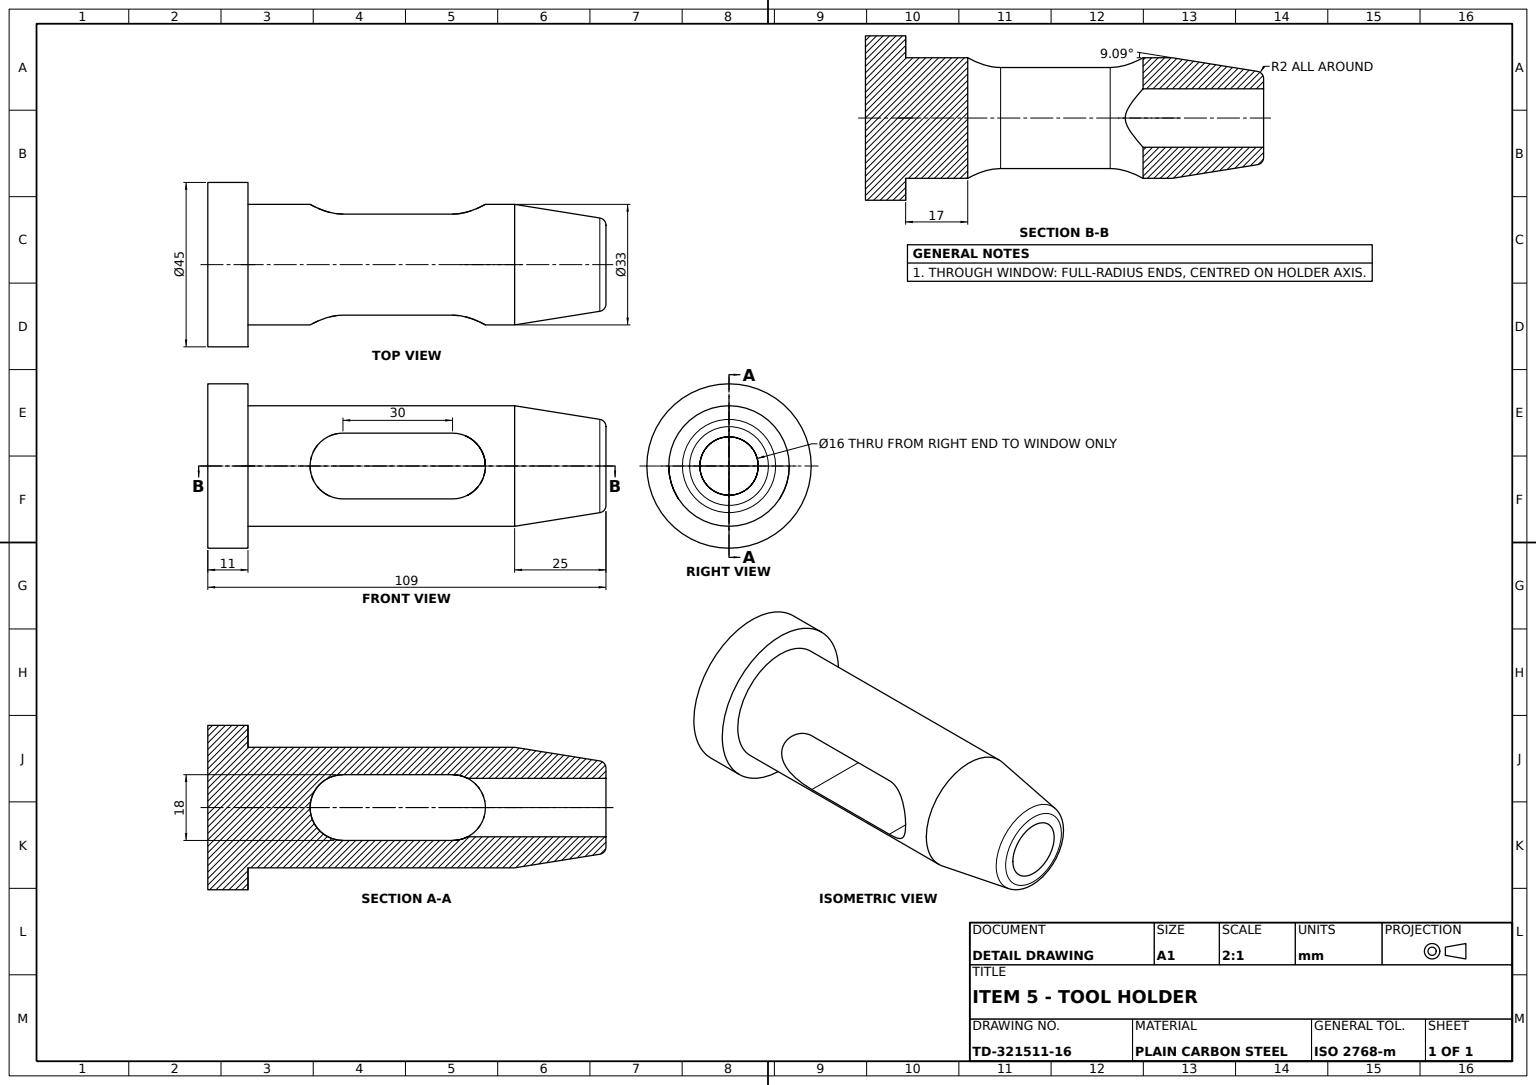
ISO-10303-21;
HEADER;
FILE_DESCRIPTION((''),'2;1');
FILE_NAME('','',(''),(''),'','','');
FILE_SCHEMA(('AUTOMOTIVE_DESIGN'));
ENDSEC;
DATA;
#1=APPLICATION_CONTEXT('');
#2=PRODUCT_CONTEXT('',#1,'mechanical');
#3=PRODUCT('','','',(#2));
#4=PRODUCT_DEFINITION_FORMATION('','',#3);
#5=PRODUCT_DEFINITION_CONTEXT('',#1,'design');
#6=PRODUCT_DEFINITION('','',#4,#5);
#7=PRODUCT_DEFINITION_SHAPE('','',#6);
#8=(LENGTH_UNIT()NAMED_UNIT(*)SI_UNIT(.MILLI.,.METRE.));
#9=(NAMED_UNIT(*)PLANE_ANGLE_UNIT()SI_UNIT($,.RADIAN.));
#10=(NAMED_UNIT(*)SI_UNIT($,.STERADIAN.)SOLID_ANGLE_UNIT());
#11=UNCERTAINTY_MEASURE_WITH_UNIT(LENGTH_MEASURE(1.E-05),#8,'distance_accuracy_value','');
#12=(GEOMETRIC_REPRESENTATION_CONTEXT(3)GLOBAL_UNCERTAINTY_ASSIGNED_CONTEXT((#11))GLOBAL_UNIT_ASSIGNED_CONTEXT((#8,#9,#10))REPRESENTATION_CONTEXT('',''));
#13=CARTESIAN_POINT('',(109.,0.,-10.794562));
#14=VERTEX_POINT('',#13);
#15=CARTESIAN_POINT('',(107.315981,0.,-12.769443));
#16=VERTEX_POINT('',#15);
#17=CARTESIAN_POINT('',(107.,0.,-10.794562));
#18=DIRECTION('',(0.,1.,0.));
#19=DIRECTION('',(0.,0.,1.));
#20=AXIS2_PLACEMENT_3D('',#17,#18,#19);
#21=CIRCLE('',#20,2.);
#22=EDGE_CURVE('',#14,#16,#21,.T.);
#23=ORIENTED_EDGE('',*,*,#22,.T.);
#24=CARTESIAN_POINT('',(107.315981,0.,12.769443));
#25=VERTEX_POINT('',#24);
#26=CARTESIAN_POINT('',(107.315981,0.,0.));
#27=DIRECTION('',(-1.,0.,0.));
#28=DIRECTION('',(0.,0.,-1.));
#29=AXIS2_PLACEMENT_3D('',#26,#27,#28);
#30=CIRCLE('',#29,12.769443);
#31=EDGE_CURVE('',#25,#16,#30,.T.);
#32=ORIENTED_EDGE('',*,*,#31,.F.);
#33=CARTESIAN_POINT('',(109.,0.,10.794562));
#34=VERTEX_POINT('',#33);
#35=CARTESIAN_POINT('',(107.,0.,10.794562));
#36=DIRECTION('',(0.,-1.,0.));
#37=AXIS2_PLACEMENT_3D('',#35,#36,#28);
#38=CIRCLE('',#37,2.);
#39=EDGE_CURVE('',#34,#25,#38,.T.);
#40=ORIENTED_EDGE('',*,*,#39,.F.);
#41=CARTESIAN_POINT('',(109.,0.,0.));
#42=DIRECTION('',(1.,0.,0.));
#43=AXIS2_PLACEMENT_3D('',#41,#42,#19);
#44=CIRCLE('',#43,10.794562);
#45=EDGE_CURVE('',#14,#34,#44,.T.);
#46=ORIENTED_EDGE('',*,*,#45,.F.);
#47=EDGE_LOOP('',(#23,#32,#40,#46));
#48=FACE_OUTER_BOUND('',#47,.T.);
#49=CARTESIAN_POINT('',(107.,0.,0.));
#50=AXIS2_PLACEMENT_3D('',#49,#27,#19);
#51=TOROIDAL_SURFACE('',#50,10.794562,2.);
#52=ADVANCED_FACE('',(#48),#51,.T.);
#53=CARTESIAN_POINT('',(67.,9.,-13.829317));
#54=VERTEX_POINT('',#53);
#55=CARTESIAN_POINT('',(37.,9.,-13.829317));
#56=VERTEX_POINT('',#55);
#57=CARTESIAN_POINT('',(-42.829787,9.,-13.829317));
#58=VECTOR('',#27,1000.);
#59=LINE('',#57,#58);
#60=EDGE_CURVE('',#54,#56,#59,.T.);
#61=ORIENTED_EDGE('',*,*,#60,.F.);
#62=CARTESIAN_POINT('',(67.,9.,13.829317));
#63=VERTEX_POINT('',#62);
#64=CARTESIAN_POINT('',(67.,9.,-22.5));
#65=VECTOR('',#19,1000.);
#66=LINE('',#64,#65);
#67=EDGE_CURVE('',#54,#63,#66,.T.);
#68=ORIENTED_EDGE('',*,*,#67,.T.);
#69=CARTESIAN_POINT('',(37.,9.,13.829317));
#70=VERTEX_POINT('',#69);
#71=CARTESIAN_POINT('',(-42.829787,9.,13.829317));
#72=VECTOR('',#42,1000.);
#73=LINE('',#71,#72);
#74=EDGE_CURVE('',#70,#63,#73,.T.);
#75=ORIENTED_EDGE('',*,*,#74,.F.);
#76=CARTESIAN_POINT('',(37.,9.,-22.5));
#77=LINE('',#76,#65);
#78=EDGE_CURVE('',#56,#70,#77,.T.);
#79=ORIENTED_EDGE('',*,*,#78,.F.);
#80=EDGE_LOOP('',(#61,#68,#75,#79));
#81=FACE_OUTER_BOUND('',#80,.T.);
#82=AXIS2_PLACEMENT_3D('',#76,#18,#19);
#83=PLANE('',#82);
#84=ADVANCED_FACE('',(#81),#83,.F.);
#85=CARTESIAN_POINT('',(11.,0.,22.5));
#86=VERTEX_POINT('',#85);
#87=CARTESIAN_POINT('',(0.,0.,22.5));
#88=VERTEX_POINT('',#87);
#89=CARTESIAN_POINT('',(-42.829787,0.,22.5));
#90=LINE('',#89,#58);
#91=EDGE_CURVE('',#86,#88,#90,.T.);
#92=ORIENTED_EDGE('',*,*,#91,.T.);
#93=CARTESIAN_POINT('',(0.,0.,-22.5));
#94=VERTEX_POINT('',#93);
#95=CARTESIAN_POINT('',(0.,0.,0.));
#96=AXIS2_PLACEMENT_3D('',#95,#27,#19);
#97=CIRCLE('',#96,22.5);
#98=EDGE_CURVE('',#94,#88,#97,.T.);
#99=ORIENTED_EDGE('',*,*,#98,.F.);
#100=CARTESIAN_POINT('',(11.,0.,-22.5));
#101=VERTEX_POINT('',#100);
#102=CARTESIAN_POINT('',(-42.829787,0.,-22.5));
#103=LINE('',#102,#58);
#104=EDGE_CURVE('',#101,#94,#103,.T.);
#105=ORIENTED_EDGE('',*,*,#104,.F.);
#106=CARTESIAN_POINT('',(11.,0.,0.));
#107=AXIS2_PLACEMENT_3D('',#106,#27,#19);
#108=CIRCLE('',#107,22.5);
#109=EDGE_CURVE('',#101,#86,#108,.T.);
#110=ORIENTED_EDGE('',*,*,#109,.T.);
#111=EDGE_LOOP('',(#92,#99,#105,#110));
#112=FACE_OUTER_BOUND('',#111,.T.);
#113=CARTESIAN_POINT('',(-42.829787,0.,0.));
#114=AXIS2_PLACEMENT_3D('',#113,#27,#19);
#115=CYLINDRICAL_SURFACE('',#114,22.5);
#116=ADVANCED_FACE('',(#112),#115,.T.);
#117=CARTESIAN_POINT('',(67.,-9.,13.829317));
#118=VERTEX_POINT('',#117);
#119=CARTESIAN_POINT('',(37.,-9.,13.829317));
#120=VERTEX_POINT('',#119);
#121=CARTESIAN_POINT('',(-42.829787,-9.,13.829317));
#122=LINE('',#121,#58);
#123=EDGE_CURVE('',#118,#120,#122,.T.);
#124=ORIENTED_EDGE('',*,*,#123,.F.);
#125=CARTESIAN_POINT('',(67.,-9.,-13.829317));
#126=VERTEX_POINT('',#125);
#127=CARTESIAN_POINT('',(67.,-9.,-22.5));
#128=LINE('',#127,#65);
#129=EDGE_CURVE('',#126,#118,#128,.T.);
#130=ORIENTED_EDGE('',*,*,#129,.F.);
#131=CARTESIAN_POINT('',(37.,-9.,-13.829317));
#132=VERTEX_POINT('',#131);
#133=CARTESIAN_POINT('',(-42.829787,-9.,-13.829317));
#134=LINE('',#133,#72);
#135=EDGE_CURVE('',#132,#126,#134,.T.);
#136=ORIENTED_EDGE('',*,*,#135,.F.);
#137=CARTESIAN_POINT('',(37.,-9.,-22.5));
#138=LINE('',#137,#65);
#139=EDGE_CURVE('',#132,#120,#138,.T.);
#140=ORIENTED_EDGE('',*,*,#139,.T.);
#141=EDGE_LOOP('',(#124,#130,#136,#140));
#142=FACE_OUTER_BOUND('',#141,.T.);
#143=AXIS2_PLACEMENT_3D('',#137,#36,#28);
#144=PLANE('',#143);
#145=ADVANCED_FACE('',(#142),#144,.F.);
#146=ORIENTED_EDGE('',*,*,#135,.T.);
#147=CARTESIAN_POINT('',(76.,0.,-16.5));
#148=VERTEX_POINT('',#147);
#149=CARTESIAN_POINT('',(67.608745,-9.,-13.829317));
#150=CARTESIAN_POINT('',(68.204136,-8.938913,-13.869585));
#151=CARTESIAN_POINT('',(69.370567,-8.702558,-14.019095));
#152=CARTESIAN_POINT('',(69.946767,-8.524146,-14.130046));
#153=CARTESIAN_POINT('',(71.028904,-8.069227,-14.39468));
#154=CARTESIAN_POINT('',(71.540157,-7.792772,-14.548404));
#155=CARTESIAN_POINT('',(72.508177,-7.14145,-14.878947));
#156=CARTESIAN_POINT('',(72.954194,-6.773387,-15.052097));
#157=CARTESIAN_POINT('',(73.564861,-6.16323,-15.307292));
#158=CARTESIAN_POINT('',(73.758993,-5.949812,-15.391775));
#159=CARTESIAN_POINT('',(74.12832,-5.501936,-15.557497));
#160=CARTESIAN_POINT('',(74.304059,-5.266458,-15.639015));
#161=CARTESIAN_POINT('',(74.791958,-4.541454,-15.870812));
#162=CARTESIAN_POINT('',(75.068713,-4.029999,-16.009872));
#163=CARTESIAN_POINT('',(75.410231,-3.217805,-16.185563));
#164=CARTESIAN_POINT('',(75.511702,-2.939521,-16.23864));
#165=CARTESIAN_POINT('',(75.688431,-2.366649,-16.331969));
#166=CARTESIAN_POINT('',(75.762616,-2.075008,-16.371651));
#167=CARTESIAN_POINT('',(75.939961,-1.197281,-16.467027));
#168=CARTESIAN_POINT('',(76.,-0.603261,-16.5));
#169=B_SPLINE_CURVE_WITH_KNOTS('',3,(#125,#149,#150,#151,#152,#153,#154,#155,#156,#157,#158,#159,#160,#161,#162,#163,#164,#165,#166,#167,#168,#147),.UNSPECIFIED.,.F.,.F.,(4,2,2,2,2,2,2,2,2,2,4),(0.,0.00179654,0.003593081,0.005389621,0.007186162,0.008084432,0.008982702,0.010779243,0.011677513,0.012575783,0.014372324),.UNSPECIFIED.);
#170=EDGE_CURVE('',#126,#148,#169,.T.);
#171=ORIENTED_EDGE('',*,*,#170,.T.);
#172=CARTESIAN_POINT('',(84.,0.,-16.5));
#173=VERTEX_POINT('',#172);
#174=CARTESIAN_POINT('',(-42.829787,0.,-16.5));
#175=LINE('',#174,#58);
#176=EDGE_CURVE('',#173,#148,#175,.T.);
#177=ORIENTED_EDGE('',*,*,#176,.F.);
#178=CARTESIAN_POINT('',(84.,0.,16.5));
#179=VERTEX_POINT('',#178);
#180=CARTESIAN_POINT('',(84.,0.,0.));
#181=AXIS2_PLACEMENT_3D('',#180,#27,#19);
#182=CIRCLE('',#181,16.5);
#183=EDGE_CURVE('',#173,#179,#182,.T.);
#184=ORIENTED_EDGE('',*,*,#183,.T.);
#185=CARTESIAN_POINT('',(76.,0.,16.5));
#186=VERTEX_POINT('',#185);
#187=CARTESIAN_POINT('',(-42.829787,0.,16.5));
#188=LINE('',#187,#58);
#189=EDGE_CURVE('',#179,#186,#188,.T.);
#190=ORIENTED_EDGE('',*,*,#189,.T.);
#191=CARTESIAN_POINT('',(76.,-0.301003,16.5));
#192=CARTESIAN_POINT('',(75.984626,-0.605798,16.4916));
#193=CARTESIAN_POINT('',(75.924121,-1.204388,16.458715));
#194=CARTESIAN_POINT('',(75.879136,-1.499868,16.434311));
#195=CARTESIAN_POINT('',(75.760581,-2.08348,16.370561));
#196=CARTESIAN_POINT('',(75.687009,-2.371611,16.331214));
#197=CARTESIAN_POINT('',(75.511256,-2.94061,16.238408));
#198=CARTESIAN_POINT('',(75.408495,-3.222513,16.184656));
#199=CARTESIAN_POINT('',(75.064128,-4.039723,16.007542));
#200=CARTESIAN_POINT('',(74.78564,-4.55228,15.8677));
#201=CARTESIAN_POINT('',(74.296702,-5.276648,15.635577));
#202=CARTESIAN_POINT('',(74.120962,-5.511434,15.554126));
#203=CARTESIAN_POINT('',(73.751604,-5.958175,15.388532));
#204=CARTESIAN_POINT('',(73.557493,-6.17105,15.304134));
#205=CARTESIAN_POINT('',(72.946994,-6.77964,15.049251));
#206=CARTESIAN_POINT('',(72.501067,-7.146844,14.876331));
#207=CARTESIAN_POINT('',(71.534185,-7.796171,14.546557));
#208=CARTESIAN_POINT('',(71.025012,-8.070838,14.39374));
#209=CARTESIAN_POINT('',(70.219751,-8.409399,14.196798));
#210=CARTESIAN_POINT('',(69.944361,-8.509905,14.13655));
#211=CARTESIAN_POINT('',(69.378428,-8.685092,14.029601));
#212=CARTESIAN_POINT('',(69.086245,-8.759986,13.982762));
#213=CARTESIAN_POINT('',(68.205376,-8.939025,13.869527));
#214=CARTESIAN_POINT('',(67.608073,-9.,13.829317));
#215=B_SPLINE_CURVE_WITH_KNOTS('',3,(#185,#191,#192,#193,#194,#195,#196,#197,#198,#199,#200,#201,#202,#203,#204,#205,#206,#207,#208,#209,#210,#211,#212,#213,#214,#117),.UNSPECIFIED.,.F.,.F.,(4,2,2,2,2,2,2,2,2,2,2,2,4),(0.014372324,0.015268727,0.016165129,0.017061532,0.017957935,0.01975074,0.020647142,0.021543545,0.02333635,0.025129156,0.026025558,0.026921961,0.028714766),.UNSPECIFIED.);
#216=EDGE_CURVE('',#186,#118,#215,.T.);
#217=ORIENTED_EDGE('',*,*,#216,.T.);
#218=ORIENTED_EDGE('',*,*,#123,.T.);
#219=CARTESIAN_POINT('',(28.,0.,16.5));
#220=VERTEX_POINT('',#219);
#221=CARTESIAN_POINT('',(36.391255,-9.,13.829317));
#222=CARTESIAN_POINT('',(35.795864,-8.938913,13.869585));
#223=CARTESIAN_POINT('',(34.629433,-8.702558,14.019095));
#224=CARTESIAN_POINT('',(34.053233,-8.524146,14.130046));
#225=CARTESIAN_POINT('',(32.971096,-8.069227,14.39468));
#226=CARTESIAN_POINT('',(32.459843,-7.792772,14.548404));
#227=CARTESIAN_POINT('',(31.491823,-7.14145,14.878947));
#228=CARTESIAN_POINT('',(31.045806,-6.773387,15.052097));
#229=CARTESIAN_POINT('',(30.435139,-6.16323,15.307292));
#230=CARTESIAN_POINT('',(30.241007,-5.949812,15.391775));
#231=CARTESIAN_POINT('',(29.87168,-5.501936,15.557497));
#232=CARTESIAN_POINT('',(29.695941,-5.266458,15.639015));
#233=CARTESIAN_POINT('',(29.208042,-4.541454,15.870812));
#234=CARTESIAN_POINT('',(28.931287,-4.029999,16.009872));
#235=CARTESIAN_POINT('',(28.589769,-3.217805,16.185563));
#236=CARTESIAN_POINT('',(28.488298,-2.939521,16.23864));
#237=CARTESIAN_POINT('',(28.311569,-2.366649,16.331969));
#238=CARTESIAN_POINT('',(28.237384,-2.075008,16.371651));
#239=CARTESIAN_POINT('',(28.060039,-1.197281,16.467027));
#240=CARTESIAN_POINT('',(28.,-0.603261,16.5));
#241=B_SPLINE_CURVE_WITH_KNOTS('',3,(#119,#221,#222,#223,#224,#225,#226,#227,#228,#229,#230,#231,#232,#233,#234,#235,#236,#237,#238,#239,#240,#219),.UNSPECIFIED.,.F.,.F.,(4,2,2,2,2,2,2,2,2,2,4),(0.,0.00179654,0.003593081,0.005389621,0.007186162,0.008084432,0.008982702,0.010779243,0.011677513,0.012575783,0.014372324),.UNSPECIFIED.);
#242=EDGE_CURVE('',#120,#220,#241,.T.);
#243=ORIENTED_EDGE('',*,*,#242,.T.);
#244=CARTESIAN_POINT('',(11.,0.,16.5));
#245=VERTEX_POINT('',#244);
#246=EDGE_CURVE('',#220,#245,#188,.T.);
#247=ORIENTED_EDGE('',*,*,#246,.T.);
#248=CARTESIAN_POINT('',(11.,0.,-16.5));
#249=VERTEX_POINT('',#248);
#250=CIRCLE('',#107,16.5);
#251=EDGE_CURVE('',#249,#245,#250,.T.);
#252=ORIENTED_EDGE('',*,*,#251,.F.);
#253=CARTESIAN_POINT('',(28.,0.,-16.5));
#254=VERTEX_POINT('',#253);
#255=EDGE_CURVE('',#254,#249,#175,.T.);
#256=ORIENTED_EDGE('',*,*,#255,.F.);
#257=CARTESIAN_POINT('',(28.,-0.301003,-16.5));
#258=CARTESIAN_POINT('',(28.015374,-0.605798,-16.4916));
#259=CARTESIAN_POINT('',(28.075879,-1.204388,-16.458715));
#260=CARTESIAN_POINT('',(28.120864,-1.499868,-16.434311));
#261=CARTESIAN_POINT('',(28.239419,-2.08348,-16.370561));
#262=CARTESIAN_POINT('',(28.312991,-2.371611,-16.331214));
#263=CARTESIAN_POINT('',(28.488744,-2.94061,-16.238408));
#264=CARTESIAN_POINT('',(28.591505,-3.222513,-16.184656));
#265=CARTESIAN_POINT('',(28.935872,-4.039723,-16.007542));
#266=CARTESIAN_POINT('',(29.21436,-4.55228,-15.8677));
#267=CARTESIAN_POINT('',(29.703298,-5.276648,-15.635577));
#268=CARTESIAN_POINT('',(29.879038,-5.511434,-15.554126));
#269=CARTESIAN_POINT('',(30.248396,-5.958175,-15.388532));
#270=CARTESIAN_POINT('',(30.442507,-6.17105,-15.304134));
#271=CARTESIAN_POINT('',(31.053006,-6.77964,-15.049251));
#272=CARTESIAN_POINT('',(31.498933,-7.146844,-14.876331));
#273=CARTESIAN_POINT('',(32.465815,-7.796171,-14.546557));
#274=CARTESIAN_POINT('',(32.974988,-8.070838,-14.39374));
#275=CARTESIAN_POINT('',(33.780249,-8.409399,-14.196798));
#276=CARTESIAN_POINT('',(34.055639,-8.509905,-14.13655));
#277=CARTESIAN_POINT('',(34.621572,-8.685092,-14.029601));
#278=CARTESIAN_POINT('',(34.913755,-8.759986,-13.982762));
#279=CARTESIAN_POINT('',(35.794624,-8.939025,-13.869527));
#280=CARTESIAN_POINT('',(36.391927,-9.,-13.829317));
#281=B_SPLINE_CURVE_WITH_KNOTS('',3,(#253,#257,#258,#259,#260,#261,#262,#263,#264,#265,#266,#267,#268,#269,#270,#271,#272,#273,#274,#275,#276,#277,#278,#279,#280,#131),.UNSPECIFIED.,.F.,.F.,(4,2,2,2,2,2,2,2,2,2,2,2,4),(0.014372324,0.015268727,0.016165129,0.017061532,0.017957935,0.01975074,0.020647142,0.021543545,0.02333635,0.025129156,0.026025558,0.026921961,0.028714766),.UNSPECIFIED.);
#282=EDGE_CURVE('',#254,#132,#281,.T.);
#283=ORIENTED_EDGE('',*,*,#282,.T.);
#284=EDGE_LOOP('',(#146,#171,#177,#184,#190,#217,#218,#243,#247,#252,#256,#283));
#285=FACE_OUTER_BOUND('',#284,.T.);
#286=CYLINDRICAL_SURFACE('',#114,16.5);
#287=ADVANCED_FACE('',(#285),#286,.T.);
#288=ORIENTED_EDGE('',*,*,#183,.F.);
#289=CARTESIAN_POINT('',(109.,0.,-12.5));
#290=DIRECTION('',(-0.987440632,0.,-0.157990501));
#291=VECTOR('',#290,1000.);
#292=LINE('',#289,#291);
#293=EDGE_CURVE('',#16,#173,#292,.T.);
#294=ORIENTED_EDGE('',*,*,#293,.F.);
#295=EDGE_CURVE('',#16,#25,#30,.T.);
#296=ORIENTED_EDGE('',*,*,#295,.T.);
#297=CARTESIAN_POINT('',(109.,0.,12.5));
#298=DIRECTION('',(-0.987440632,0.,0.157990501));
#299=VECTOR('',#298,1000.);
#300=LINE('',#297,#299);
#301=EDGE_CURVE('',#25,#179,#300,.T.);
#302=ORIENTED_EDGE('',*,*,#301,.T.);
#303=EDGE_LOOP('',(#288,#294,#296,#302));
#304=FACE_OUTER_BOUND('',#303,.T.);
#305=AXIS2_PLACEMENT_3D('',#41,#27,#19);
#306=CONICAL_SURFACE('',#305,12.5,0.158655262);
#307=ADVANCED_FACE('',(#304),#306,.T.);
#308=EDGE_CURVE('',#88,#94,#97,.T.);
#309=ORIENTED_EDGE('',*,*,#308,.T.);
#310=ORIENTED_EDGE('',*,*,#98,.T.);
#311=EDGE_LOOP('',(#309,#310));
#312=FACE_OUTER_BOUND('',#311,.T.);
#313=AXIS2_PLACEMENT_3D('',#95,#42,#28);
#314=PLANE('',#313);
#315=ADVANCED_FACE('',(#312),#314,.F.);
#316=CARTESIAN_POINT('',(76.,0.,8.));
#317=VERTEX_POINT('',#316);
#318=CARTESIAN_POINT('',(109.,0.,8.));
#319=VERTEX_POINT('',#318);
#320=CARTESIAN_POINT('',(-0.001,0.,8.));
#321=LINE('',#320,#72);
#322=EDGE_CURVE('',#317,#319,#321,.T.);
#323=ORIENTED_EDGE('',*,*,#322,.F.);
#324=CARTESIAN_POINT('',(76.,0.,-8.));
#325=VERTEX_POINT('',#324);
#326=CARTESIAN_POINT('',(76.,0.283229,8.));
#327=CARTESIAN_POINT('',(75.98643,0.570141,7.984743));
#328=CARTESIAN_POINT('',(75.932459,1.136736,7.923952));
#329=CARTESIAN_POINT('',(75.892481,1.41449,7.878894));
#330=CARTESIAN_POINT('',(75.788444,1.959657,7.761282));
#331=CARTESIAN_POINT('',(75.724377,2.227066,7.688721));
#332=CARTESIAN_POINT('',(75.573303,2.751916,7.516862));
#333=CARTESIAN_POINT('',(75.486786,3.007241,7.418113));
#334=CARTESIAN_POINT('',(75.296896,3.497221,7.200094));
#335=CARTESIAN_POINT('',(75.193148,3.733175,7.0804));
#336=CARTESIAN_POINT('',(74.969998,4.188486,6.820942));
#337=CARTESIAN_POINT('',(74.849921,4.408881,6.680382));
#338=CARTESIAN_POINT('',(74.474441,5.036934,6.236364));
#339=CARTESIAN_POINT('',(74.204096,5.412659,5.911262));
#340=CARTESIAN_POINT('',(73.779744,5.923179,5.38293));
#341=CARTESIAN_POINT('',(73.635127,6.084405,5.199952));
#342=CARTESIAN_POINT('',(73.34149,6.389866,4.819657));
#343=CARTESIAN_POINT('',(73.192093,6.534364,4.621807));
#344=CARTESIAN_POINT('',(72.747943,6.936919,4.01437));
#345=CARTESIAN_POINT('',(72.454337,7.16683,3.588994));
#346=CARTESIAN_POINT('',(72.041518,7.457306,2.906832));
#347=CARTESIAN_POINT('',(71.908647,7.54498,2.671966));
#348=CARTESIAN_POINT('',(71.66006,7.700998,2.181914));
#349=CARTESIAN_POINT('',(71.544431,7.769226,1.926362));
#350=CARTESIAN_POINT('',(71.348299,7.880674,1.402399));
#351=CARTESIAN_POINT('',(71.266953,7.924471,1.132487));
#352=CARTESIAN_POINT('',(71.153337,7.984605,0.570831));
#353=CARTESIAN_POINT('',(71.123423,7.999836,0.287616));
#354=CARTESIAN_POINT('',(71.122951,8.00008,-0.136931));
#355=CARTESIAN_POINT('',(71.130098,7.996409,-0.278613));
#356=CARTESIAN_POINT('',(71.158879,7.981478,-0.562307));
#357=CARTESIAN_POINT('',(71.180733,7.970099,-0.705178));
#358=CARTESIAN_POINT('',(71.264904,7.925568,-1.12445));
#359=CARTESIAN_POINT('',(71.345498,7.882208,-1.39367));
#360=CARTESIAN_POINT('',(71.540469,7.771532,-1.916983));
#361=CARTESIAN_POINT('',(71.655674,7.703644,-2.172564));
#362=CARTESIAN_POINT('',(71.903734,7.548167,-2.662957));
#363=CARTESIAN_POINT('',(72.036564,7.460655,-2.898273));
#364=CARTESIAN_POINT('',(72.44988,7.170232,-3.582353));
#365=CARTESIAN_POINT('',(72.74466,6.939769,-4.009789));
#366=CARTESIAN_POINT('',(73.34034,6.400125,-4.824645));
#367=CARTESIAN_POINT('',(73.635195,6.096741,-5.202883));
#368=CARTESIAN_POINT('',(74.060005,5.586175,-5.731903));
#369=CARTESIAN_POINT('',(74.198759,5.406671,-5.901741));
#370=CARTESIAN_POINT('',(74.468704,5.027193,-6.228159));
#371=CARTESIAN_POINT('',(74.600531,4.826124,-6.385477));
#372=CARTESIAN_POINT('',(74.97605,4.197715,-6.829519));
#373=CARTESIAN_POINT('',(75.200044,3.746365,-7.08888));
#374=CARTESIAN_POINT('',(75.485178,3.011768,-7.416274));
#375=CARTESIAN_POINT('',(75.572176,2.755346,-7.515575));
#376=CARTESIAN_POINT('',(75.723057,2.232131,-7.687223));
#377=CARTESIAN_POINT('',(75.787185,1.965268,-7.759857));
#378=CARTESIAN_POINT('',(75.943671,1.148194,-7.936767));
#379=CARTESIAN_POINT('',(76.,0.575822,-8.));
#380=B_SPLINE_CURVE_WITH_KNOTS('',3,(#316,#326,#327,#328,#329,#330,#331,#332,#333,#334,#335,#336,#337,#338,#339,#340,#341,#342,#343,#344,#345,#346,#347,#348,#349,#350,#351,#352,#353,#354,#355,#356,#357,#358,#359,#360,#361,#362,#363,#364,#365,#366,#367,#368,#369,#370,#371,#372,#373,#374,#375,#376,#377,#378,#379,#324),.UNSPECIFIED.,.F.,.F.,(4,2,2,2,2,2,2,2,2,2,2,2,2,2,2,2,2,2,2,2,2,2,2,2,2,2,2,4),(0.027190861,0.028040032,0.028889203,0.029738373,0.030587544,0.031436715,0.032285886,0.033984227,0.034833398,0.035682568,0.03738091,0.038230081,0.039079251,0.039928422,0.040777593,0.041202178,0.041626763,0.042475934,0.043325105,0.044174276,0.045872617,0.047570958,0.048420129,0.0492693,0.050967641,0.051816812,0.052665983,0.054364324),.UNSPECIFIED.);
#381=EDGE_CURVE('',#317,#325,#380,.T.);
#382=ORIENTED_EDGE('',*,*,#381,.T.);
#383=CARTESIAN_POINT('',(109.,0.,-8.));
#384=VERTEX_POINT('',#383);
#385=CARTESIAN_POINT('',(-0.001,0.,-8.));
#386=LINE('',#385,#72);
#387=EDGE_CURVE('',#325,#384,#386,.T.);
#388=ORIENTED_EDGE('',*,*,#387,.T.);
#389=AXIS2_PLACEMENT_3D('',#41,#42,#28);
#390=CIRCLE('',#389,8.);
#391=EDGE_CURVE('',#384,#319,#390,.T.);
#392=ORIENTED_EDGE('',*,*,#391,.T.);
#393=EDGE_LOOP('',(#323,#382,#388,#392));
#394=FACE_OUTER_BOUND('',#393,.T.);
#395=CARTESIAN_POINT('',(-0.001,0.,0.));
#396=AXIS2_PLACEMENT_3D('',#395,#42,#28);
#397=CYLINDRICAL_SURFACE('',#396,8.);
#398=ADVANCED_FACE('',(#394),#397,.F.);
#399=ORIENTED_EDGE('',*,*,#216,.F.);
#400=CARTESIAN_POINT('',(76.,0.,-22.5));
#401=LINE('',#400,#65);
#402=EDGE_CURVE('',#317,#186,#401,.T.);
#403=ORIENTED_EDGE('',*,*,#402,.F.);
#404=CARTESIAN_POINT('',(76.,-0.576191,-8.));
#405=CARTESIAN_POINT('',(75.945227,-1.137067,-7.93852));
#406=CARTESIAN_POINT('',(75.788956,-1.957487,-7.761862));
#407=CARTESIAN_POINT('',(75.723796,-2.229291,-7.688062));
#408=CARTESIAN_POINT('',(75.572832,-2.753343,-7.516324));
#409=CARTESIAN_POINT('',(75.4871,-3.006337,-7.418472));
#410=CARTESIAN_POINT('',(75.297426,-3.495947,-7.200704));
#411=CARTESIAN_POINT('',(75.193475,-3.732556,-7.080781));
#412=CARTESIAN_POINT('',(74.969025,-4.190422,-6.819809));
#413=CARTESIAN_POINT('',(74.849019,-4.410437,-6.679319));
#414=CARTESIAN_POINT('',(74.474849,-5.036155,-6.236839));
#415=CARTESIAN_POINT('',(74.204361,-5.412473,-5.911625));
#416=CARTESIAN_POINT('',(73.635799,-6.096217,-5.203683));
#417=CARTESIAN_POINT('',(73.336258,-6.403968,-4.819166));
#418=CARTESIAN_POINT('',(72.745136,-6.939192,-4.010334));
#419=CARTESIAN_POINT('',(72.450746,-7.16966,-3.58389));
#420=CARTESIAN_POINT('',(72.035129,-7.461645,-2.895847));
#421=CARTESIAN_POINT('',(71.900536,-7.550241,-2.657102));
#422=CARTESIAN_POINT('',(71.65257,-7.705517,-2.165951));
#423=CARTESIAN_POINT('',(71.538782,-7.77252,-1.91314));
#424=CARTESIAN_POINT('',(71.343421,-7.883356,-1.387396));
#425=CARTESIAN_POINT('',(71.261951,-7.927147,-1.112807));
#426=CARTESIAN_POINT('',(71.151681,-7.985452,-0.557282));
#427=CARTESIAN_POINT('',(71.122113,-8.000511,-0.273909));
#428=CARTESIAN_POINT('',(71.124149,-7.999462,0.303014));
#429=CARTESIAN_POINT('',(71.155608,-7.983424,0.585498));
#430=CARTESIAN_POINT('',(71.269262,-7.923228,1.140317));
#431=CARTESIAN_POINT('',(71.352278,-7.878485,1.414585));
#432=CARTESIAN_POINT('',(71.647826,-7.710325,2.199359));
#433=CARTESIAN_POINT('',(71.905528,-7.553276,2.682879));
#434=CARTESIAN_POINT('',(72.46277,-7.160609,3.602151));
#435=CARTESIAN_POINT('',(72.757058,-6.929213,4.027234));
#436=CARTESIAN_POINT('',(73.345,-6.395208,4.83052));
#437=CARTESIAN_POINT('',(73.639335,-6.092591,5.208231));
#438=CARTESIAN_POINT('',(74.211223,-5.403583,5.920019));
#439=CARTESIAN_POINT('',(74.482529,-5.024551,6.246013));
#440=CARTESIAN_POINT('',(74.854382,-4.400826,6.685613));
#441=CARTESIAN_POINT('',(74.97264,-4.183467,6.824028));
#442=CARTESIAN_POINT('',(75.195684,-3.727619,7.083333));
#443=CARTESIAN_POINT('',(75.300767,-3.488051,7.204554));
#444=CARTESIAN_POINT('',(75.585172,-2.751683,7.531043));
#445=CARTESIAN_POINT('',(75.736626,-2.233036,7.702707));
#446=CARTESIAN_POINT('',(75.893947,-1.405874,7.880549));
#447=CARTESIAN_POINT('',(75.933739,-1.125865,7.925395));
#448=CARTESIAN_POINT('',(75.986643,-0.565255,7.984982));
#449=CARTESIAN_POINT('',(76.,-0.283411,8.));
#450=B_SPLINE_CURVE_WITH_KNOTS('',3,(#324,#404,#405,#406,#407,#408,#409,#410,#411,#412,#413,#414,#415,#416,#417,#418,#419,#420,#421,#422,#423,#424,#425,#426,#427,#428,#429,#430,#431,#432,#433,#434,#435,#436,#437,#438,#439,#440,#441,#442,#443,#444,#445,#446,#447,#448,#449,#316),.UNSPECIFIED.,.F.,.F.,(4,2,2,2,2,2,2,2,2,2,2,2,2,2,2,2,2,2,2,2,2,2,2,4),(0.,0.001699429,0.002549143,0.003398858,0.004248572,0.005098286,0.006797715,0.008497144,0.010196573,0.011046287,0.011896002,0.012745716,0.013595431,0.014445145,0.015294859,0.016994288,0.018693717,0.020393146,0.022092575,0.022942289,0.023792004,0.025491432,0.026341147,0.027190861),.UNSPECIFIED.);
#451=EDGE_CURVE('',#325,#317,#450,.T.);
#452=ORIENTED_EDGE('',*,*,#451,.F.);
#453=EDGE_CURVE('',#148,#325,#401,.T.);
#454=ORIENTED_EDGE('',*,*,#453,.F.);
#455=ORIENTED_EDGE('',*,*,#170,.F.);
#456=ORIENTED_EDGE('',*,*,#129,.T.);
#457=EDGE_LOOP('',(#399,#403,#452,#454,#455,#456));
#458=FACE_OUTER_BOUND('',#457,.T.);
#459=CARTESIAN_POINT('',(67.,0.,-22.5));
#460=AXIS2_PLACEMENT_3D('',#459,#19,#42);
#461=CYLINDRICAL_SURFACE('',#460,9.);
#462=ADVANCED_FACE('',(#458),#461,.F.);
#463=ORIENTED_EDGE('',*,*,#31,.T.);
#464=ORIENTED_EDGE('',*,*,#293,.T.);
#465=EDGE_CURVE('',#179,#173,#182,.T.);
#466=ORIENTED_EDGE('',*,*,#465,.F.);
#467=ORIENTED_EDGE('',*,*,#301,.F.);
#468=EDGE_LOOP('',(#463,#464,#466,#467));
#469=FACE_OUTER_BOUND('',#468,.T.);
#470=ADVANCED_FACE('',(#469),#306,.T.);
#471=EDGE_CURVE('',#34,#14,#44,.T.);
#472=ORIENTED_EDGE('',*,*,#471,.T.);
#473=ORIENTED_EDGE('',*,*,#45,.T.);
#474=EDGE_LOOP('',(#472,#473));
#475=FACE_OUTER_BOUND('',#474,.T.);
#476=ORIENTED_EDGE('',*,*,#391,.F.);
#477=EDGE_CURVE('',#319,#384,#390,.T.);
#478=ORIENTED_EDGE('',*,*,#477,.F.);
#479=EDGE_LOOP('',(#476,#478));
#480=FACE_BOUND('',#479,.T.);
#481=CARTESIAN_POINT('',(109.,12.5,0.));
#482=AXIS2_PLACEMENT_3D('',#481,#27,#19);
#483=PLANE('',#482);
#484=ADVANCED_FACE('',(#475,#480),#483,.F.);
#485=ORIENTED_EDGE('',*,*,#242,.F.);
#486=ORIENTED_EDGE('',*,*,#139,.F.);
#487=ORIENTED_EDGE('',*,*,#282,.F.);
#488=CARTESIAN_POINT('',(36.391255,9.,-13.829317));
#489=CARTESIAN_POINT('',(35.795864,8.938913,-13.869585));
#490=CARTESIAN_POINT('',(34.629433,8.702558,-14.019095));
#491=CARTESIAN_POINT('',(34.053233,8.524146,-14.130046));
#492=CARTESIAN_POINT('',(32.971096,8.069227,-14.39468));
#493=CARTESIAN_POINT('',(32.459843,7.792772,-14.548404));
#494=CARTESIAN_POINT('',(31.491823,7.14145,-14.878947));
#495=CARTESIAN_POINT('',(31.045806,6.773387,-15.052097));
#496=CARTESIAN_POINT('',(30.435139,6.16323,-15.307292));
#497=CARTESIAN_POINT('',(30.241007,5.949812,-15.391775));
#498=CARTESIAN_POINT('',(29.87168,5.501936,-15.557497));
#499=CARTESIAN_POINT('',(29.695941,5.266458,-15.639015));
#500=CARTESIAN_POINT('',(29.208042,4.541454,-15.870812));
#501=CARTESIAN_POINT('',(28.931287,4.029999,-16.009872));
#502=CARTESIAN_POINT('',(28.589769,3.217805,-16.185563));
#503=CARTESIAN_POINT('',(28.488298,2.939521,-16.23864));
#504=CARTESIAN_POINT('',(28.311569,2.366649,-16.331969));
#505=CARTESIAN_POINT('',(28.237384,2.075008,-16.371651));
#506=CARTESIAN_POINT('',(28.060039,1.197281,-16.467027));
#507=CARTESIAN_POINT('',(28.,0.603261,-16.5));
#508=B_SPLINE_CURVE_WITH_KNOTS('',3,(#55,#488,#489,#490,#491,#492,#493,#494,#495,#496,#497,#498,#499,#500,#501,#502,#503,#504,#505,#506,#507,#253),.UNSPECIFIED.,.F.,.F.,(4,2,2,2,2,2,2,2,2,2,4),(0.,0.00179654,0.003593081,0.005389621,0.007186162,0.008084432,0.008982702,0.010779243,0.011677513,0.012575783,0.014372324),.UNSPECIFIED.);
#509=EDGE_CURVE('',#56,#254,#508,.T.);
#510=ORIENTED_EDGE('',*,*,#509,.F.);
#511=ORIENTED_EDGE('',*,*,#78,.T.);
#512=CARTESIAN_POINT('',(28.,0.301003,16.5));
#513=CARTESIAN_POINT('',(28.015374,0.605798,16.4916));
#514=CARTESIAN_POINT('',(28.075879,1.204388,16.458715));
#515=CARTESIAN_POINT('',(28.120864,1.499868,16.434311));
#516=CARTESIAN_POINT('',(28.239419,2.08348,16.370561));
#517=CARTESIAN_POINT('',(28.312991,2.371611,16.331214));
#518=CARTESIAN_POINT('',(28.488744,2.94061,16.238408));
#519=CARTESIAN_POINT('',(28.591505,3.222513,16.184656));
#520=CARTESIAN_POINT('',(28.935872,4.039723,16.007542));
#521=CARTESIAN_POINT('',(29.21436,4.55228,15.8677));
#522=CARTESIAN_POINT('',(29.703298,5.276648,15.635577));
#523=CARTESIAN_POINT('',(29.879038,5.511434,15.554126));
#524=CARTESIAN_POINT('',(30.248396,5.958175,15.388532));
#525=CARTESIAN_POINT('',(30.442507,6.17105,15.304134));
#526=CARTESIAN_POINT('',(31.053006,6.77964,15.049251));
#527=CARTESIAN_POINT('',(31.498933,7.146844,14.876331));
#528=CARTESIAN_POINT('',(32.465815,7.796171,14.546557));
#529=CARTESIAN_POINT('',(32.974988,8.070838,14.39374));
#530=CARTESIAN_POINT('',(33.780249,8.409399,14.196798));
#531=CARTESIAN_POINT('',(34.055639,8.509905,14.13655));
#532=CARTESIAN_POINT('',(34.621572,8.685092,14.029601));
#533=CARTESIAN_POINT('',(34.913755,8.759986,13.982762));
#534=CARTESIAN_POINT('',(35.794624,8.939025,13.869527));
#535=CARTESIAN_POINT('',(36.391927,9.,13.829317));
#536=B_SPLINE_CURVE_WITH_KNOTS('',3,(#219,#512,#513,#514,#515,#516,#517,#518,#519,#520,#521,#522,#523,#524,#525,#526,#527,#528,#529,#530,#531,#532,#533,#534,#535,#69),.UNSPECIFIED.,.F.,.F.,(4,2,2,2,2,2,2,2,2,2,2,2,4),(0.014372324,0.015268727,0.016165129,0.017061532,0.017957935,0.01975074,0.020647142,0.021543545,0.02333635,0.025129156,0.026025558,0.026921961,0.028714766),.UNSPECIFIED.);
#537=EDGE_CURVE('',#220,#70,#536,.T.);
#538=ORIENTED_EDGE('',*,*,#537,.F.);
#539=EDGE_LOOP('',(#485,#486,#487,#510,#511,#538));
#540=FACE_OUTER_BOUND('',#539,.T.);
#541=CARTESIAN_POINT('',(37.,0.,-22.5));
#542=AXIS2_PLACEMENT_3D('',#541,#19,#42);
#543=CYLINDRICAL_SURFACE('',#542,9.);
#544=ADVANCED_FACE('',(#540),#543,.F.);
#545=ORIENTED_EDGE('',*,*,#387,.F.);
#546=ORIENTED_EDGE('',*,*,#451,.T.);
#547=ORIENTED_EDGE('',*,*,#322,.T.);
#548=ORIENTED_EDGE('',*,*,#477,.T.);
#549=EDGE_LOOP('',(#545,#546,#547,#548));
#550=FACE_OUTER_BOUND('',#549,.T.);
#551=ADVANCED_FACE('',(#550),#397,.F.);
#552=ORIENTED_EDGE('',*,*,#22,.F.);
#553=ORIENTED_EDGE('',*,*,#471,.F.);
#554=ORIENTED_EDGE('',*,*,#39,.T.);
#555=ORIENTED_EDGE('',*,*,#295,.F.);
#556=EDGE_LOOP('',(#552,#553,#554,#555));
#557=FACE_OUTER_BOUND('',#556,.T.);
#558=ADVANCED_FACE('',(#557),#51,.T.);
#559=EDGE_CURVE('',#245,#249,#250,.T.);
#560=ORIENTED_EDGE('',*,*,#559,.F.);
#561=ORIENTED_EDGE('',*,*,#246,.F.);
#562=ORIENTED_EDGE('',*,*,#537,.T.);
#563=ORIENTED_EDGE('',*,*,#74,.T.);
#564=CARTESIAN_POINT('',(67.608745,9.,13.829317));
#565=CARTESIAN_POINT('',(68.204136,8.938913,13.869585));
#566=CARTESIAN_POINT('',(69.370567,8.702558,14.019095));
#567=CARTESIAN_POINT('',(69.946767,8.524146,14.130046));
#568=CARTESIAN_POINT('',(71.028904,8.069227,14.39468));
#569=CARTESIAN_POINT('',(71.540157,7.792772,14.548404));
#570=CARTESIAN_POINT('',(72.508177,7.14145,14.878947));
#571=CARTESIAN_POINT('',(72.954194,6.773387,15.052097));
#572=CARTESIAN_POINT('',(73.564861,6.16323,15.307292));
#573=CARTESIAN_POINT('',(73.758993,5.949812,15.391775));
#574=CARTESIAN_POINT('',(74.12832,5.501936,15.557497));
#575=CARTESIAN_POINT('',(74.304059,5.266458,15.639015));
#576=CARTESIAN_POINT('',(74.791958,4.541454,15.870812));
#577=CARTESIAN_POINT('',(75.068713,4.029999,16.009872));
#578=CARTESIAN_POINT('',(75.410231,3.217805,16.185563));
#579=CARTESIAN_POINT('',(75.511702,2.939521,16.23864));
#580=CARTESIAN_POINT('',(75.688431,2.366649,16.331969));
#581=CARTESIAN_POINT('',(75.762616,2.075008,16.371651));
#582=CARTESIAN_POINT('',(75.939961,1.197281,16.467027));
#583=CARTESIAN_POINT('',(76.,0.603261,16.5));
#584=B_SPLINE_CURVE_WITH_KNOTS('',3,(#62,#564,#565,#566,#567,#568,#569,#570,#571,#572,#573,#574,#575,#576,#577,#578,#579,#580,#581,#582,#583,#185),.UNSPECIFIED.,.F.,.F.,(4,2,2,2,2,2,2,2,2,2,4),(0.,0.00179654,0.003593081,0.005389621,0.007186162,0.008084432,0.008982702,0.010779243,0.011677513,0.012575783,0.014372324),.UNSPECIFIED.);
#585=EDGE_CURVE('',#63,#186,#584,.T.);
#586=ORIENTED_EDGE('',*,*,#585,.T.);
#587=ORIENTED_EDGE('',*,*,#189,.F.);
#588=ORIENTED_EDGE('',*,*,#465,.T.);
#589=ORIENTED_EDGE('',*,*,#176,.T.);
#590=CARTESIAN_POINT('',(76.,0.301003,-16.5));
#591=CARTESIAN_POINT('',(75.984626,0.605798,-16.4916));
#592=CARTESIAN_POINT('',(75.924121,1.204388,-16.458715));
#593=CARTESIAN_POINT('',(75.879136,1.499868,-16.434311));
#594=CARTESIAN_POINT('',(75.760581,2.08348,-16.370561));
#595=CARTESIAN_POINT('',(75.687009,2.371611,-16.331214));
#596=CARTESIAN_POINT('',(75.511256,2.94061,-16.238408));
#597=CARTESIAN_POINT('',(75.408495,3.222513,-16.184656));
#598=CARTESIAN_POINT('',(75.064128,4.039723,-16.007542));
#599=CARTESIAN_POINT('',(74.78564,4.55228,-15.8677));
#600=CARTESIAN_POINT('',(74.296702,5.276648,-15.635577));
#601=CARTESIAN_POINT('',(74.120962,5.511434,-15.554126));
#602=CARTESIAN_POINT('',(73.751604,5.958175,-15.388532));
#603=CARTESIAN_POINT('',(73.557493,6.17105,-15.304134));
#604=CARTESIAN_POINT('',(72.946994,6.77964,-15.049251));
#605=CARTESIAN_POINT('',(72.501067,7.146844,-14.876331));
#606=CARTESIAN_POINT('',(71.534185,7.796171,-14.546557));
#607=CARTESIAN_POINT('',(71.025012,8.070838,-14.39374));
#608=CARTESIAN_POINT('',(70.219751,8.409399,-14.196798));
#609=CARTESIAN_POINT('',(69.944361,8.509905,-14.13655));
#610=CARTESIAN_POINT('',(69.378428,8.685092,-14.029601));
#611=CARTESIAN_POINT('',(69.086245,8.759986,-13.982762));
#612=CARTESIAN_POINT('',(68.205376,8.939025,-13.869527));
#613=CARTESIAN_POINT('',(67.608073,9.,-13.829317));
#614=B_SPLINE_CURVE_WITH_KNOTS('',3,(#147,#590,#591,#592,#593,#594,#595,#596,#597,#598,#599,#600,#601,#602,#603,#604,#605,#606,#607,#608,#609,#610,#611,#612,#613,#53),.UNSPECIFIED.,.F.,.F.,(4,2,2,2,2,2,2,2,2,2,2,2,4),(0.014372324,0.015268727,0.016165129,0.017061532,0.017957935,0.01975074,0.020647142,0.021543545,0.02333635,0.025129156,0.026025558,0.026921961,0.028714766),.UNSPECIFIED.);
#615=EDGE_CURVE('',#148,#54,#614,.T.);
#616=ORIENTED_EDGE('',*,*,#615,.T.);
#617=ORIENTED_EDGE('',*,*,#60,.T.);
#618=ORIENTED_EDGE('',*,*,#509,.T.);
#619=ORIENTED_EDGE('',*,*,#255,.T.);
#620=EDGE_LOOP('',(#560,#561,#562,#563,#586,#587,#588,#589,#616,#617,#618,#619));
#621=FACE_OUTER_BOUND('',#620,.T.);
#622=ADVANCED_FACE('',(#621),#286,.T.);
#623=ORIENTED_EDGE('',*,*,#615,.F.);
#624=ORIENTED_EDGE('',*,*,#453,.T.);
#625=ORIENTED_EDGE('',*,*,#381,.F.);
#626=ORIENTED_EDGE('',*,*,#402,.T.);
#627=ORIENTED_EDGE('',*,*,#585,.F.);
#628=ORIENTED_EDGE('',*,*,#67,.F.);
#629=EDGE_LOOP('',(#623,#624,#625,#626,#627,#628));
#630=FACE_OUTER_BOUND('',#629,.T.);
#631=ADVANCED_FACE('',(#630),#461,.F.);
#632=ORIENTED_EDGE('',*,*,#559,.T.);
#633=ORIENTED_EDGE('',*,*,#251,.T.);
#634=EDGE_LOOP('',(#632,#633));
#635=FACE_BOUND('',#634,.T.);
#636=EDGE_CURVE('',#86,#101,#108,.T.);
#637=ORIENTED_EDGE('',*,*,#636,.F.);
#638=ORIENTED_EDGE('',*,*,#109,.F.);
#639=EDGE_LOOP('',(#637,#638));
#640=FACE_OUTER_BOUND('',#639,.T.);
#641=CARTESIAN_POINT('',(11.,22.5,0.));
#642=AXIS2_PLACEMENT_3D('',#641,#27,#19);
#643=PLANE('',#642);
#644=ADVANCED_FACE('',(#635,#640),#643,.F.);
#645=ORIENTED_EDGE('',*,*,#308,.F.);
#646=ORIENTED_EDGE('',*,*,#91,.F.);
#647=ORIENTED_EDGE('',*,*,#636,.T.);
#648=ORIENTED_EDGE('',*,*,#104,.T.);
#649=EDGE_LOOP('',(#645,#646,#647,#648));
#650=FACE_OUTER_BOUND('',#649,.T.);
#651=ADVANCED_FACE('',(#650),#115,.T.);
#652=CLOSED_SHELL('',(#52,#84,#116,#145,#287,#307,#315,#398,#462,#470,#484,#544,#551,#558,#622,#631,#644,#651));
#653=MANIFOLD_SOLID_BREP('',#652);
#654=ADVANCED_BREP_SHAPE_REPRESENTATION('',(#653),#12);
#655=SHAPE_DEFINITION_REPRESENTATION(#7,#654);
ENDSEC;
END-ISO-10303-21;
